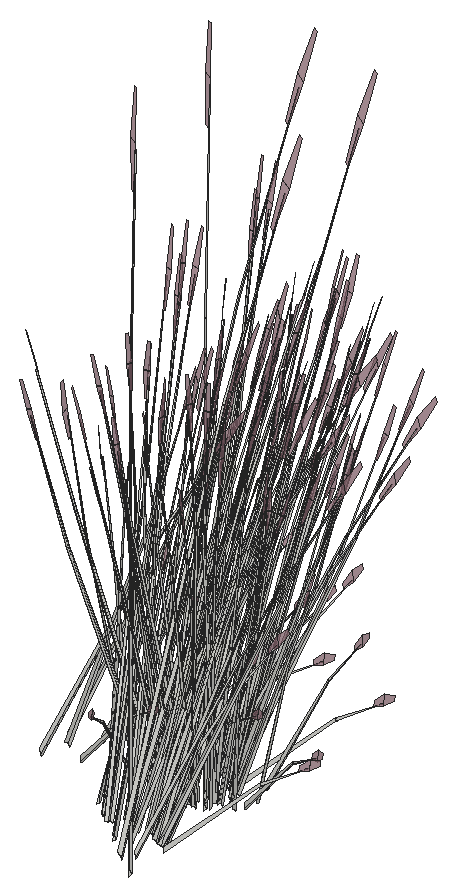
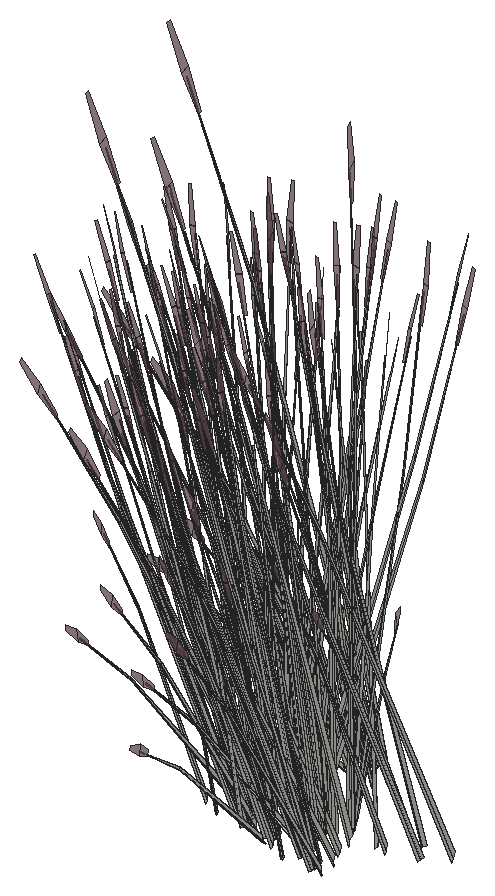
# SketchUp Ruby script. Lengths in inches.
U = 1.inch
M = Sketchup.active_model
def pt(a) = Geom::Point3d.new(a.map { |v| v * U })
def face(e, loops, mat)
  f = e.add_face(loops[0].map { |a| pt(a) })
  loops[1..].each { |l| e.add_face(l.map { |a| pt(a) }).erase! }
  f.material = f.back_material = mat if mat
  f
end
# faces: each face lists its corners as indices into pts; further lists are holes
def faces(e, pts, list, mat = nil) = list.each { |f| face(e, (f[0].is_a?(Array) ? f : [f]).map { |l| l.map { |i| pts[i] } }, mat) }
# xy, xz, yz: faces in a plane at the given z, y or x. An outline is a flat list of corners, or four numbers for a rectangle; further outlines are holes
def ring(l) = l.size == 4 ? [[l[0], l[1]], [l[2], l[1]], [l[2], l[3]], [l[0], l[3]]] : l.each_slice(2).to_a
def flat(e, list, mat, &to3) = list.each { |f| face(e, (f[0].is_a?(Array) ? f : [f]).map { |l| ring(l).map { |u, v| to3.(u, v) } }, mat) }
def xy(e, z, list, mat = nil) = flat(e, list, mat) { |x, y| [x, y, z] }
def xz(e, y, list, mat = nil) = flat(e, list, mat) { |x, z| [x, y, z] }
def yz(e, x, list, mat = nil) = flat(e, list, mat) { |y, z| [x, y, z] }
def lines(e, pts, list) = list.each { |a, b| e.add_line(pt(pts[a]), pt(pts[b])) }
# prism: a flat outline (further loops are holes) pulled along v
def prism(e, loops, v, mat = nil)
  f = face(e, loops, mat); d = Geom::Vector3d.new(v.map { |x| x * U })
  f.pushpull(f.normal.samedirection?(d) ? d.length : -d.length)
end
def box(e, o, s, mat = nil) = prism(e, [[o, [o[0] + s[0], o[1], o[2]], [o[0] + s[0], o[1] + s[1], o[2]], [o[0], o[1] + s[1], o[2]]]], [0, 0, s[2]], mat)
def at(x, y, z, deg = 0) = Geom::Transformation.translation(pt([x, y, z])) * Geom::Transformation.rotation(ORIGIN, Z_AXIS, deg.degrees)
def axes(o, x, y, z) = Geom::Transformation.new([*x, 0, *y, 0, *z, 0, *pt(o).to_a, 1])
def part(name) = M.definitions.add(name)
# library, detail: a bought-in or finely detailed component or shape, given as its bounding box
def library(name, o, s) = part(name).tap { |d| box(d.entities, o, s) }
def detail(e, o, s) = box(e.add_group.entities, o, s)
def put(e, d, t, mat = nil) = e.add_instance(d, t).tap { |i| i.material = mat if mat }
def group(e, t, mat = nil) = e.add_group.tap { |g| g.transformation = t; g.material = mat if mat }.entities
root = M.entities
M.materials.add("LightPink_Translucent").color = [144, 107, 117]
M.materials["LightPink_Translucent"].alpha = 0.75
c1 = part("blade")
p = [[2.15,0.21,22],[0,0.17,0],[0.09,0.45,0],[2.18,0.31,22],[2.29,0.31,22],[0.38,0.45,0],
  [2.48,0.24,33],[2.49,0.24,33],[2.48,0.22,33]]
faces(c1.entities,p,[[0,1,2,3],[4,5,2,3],[6,3,4,7],[8,0,3,6]])
c2 = part("seeds")
p = [[0.3,-0.1,1.38],[-0.01,-0.03,1.59],[-0.01,-0.03,0.03],[0.14,-0.07,-0.07],[0.29,-0.03,3],[0.15,0.01,3.11]]
faces(c2.entities,p,[[0,1,2,3],[1,0,4,5]],"LightPink_Translucent")
c3 = part("blade with seeds")
put(c3.entities,c1,at(0,0,0))
put(c3.entities,c2,axes([2.4,0.25,30.99],[1.5799,-0.05474,1.17369],[-0.12525,1.92788,0.29478],[-0.07173,-0.02425,1.56792]))
put(root,c3,axes([683.69,340.44,268.15],[0.46573,0.38364,-0.47077],[-0.49199,0.33598,-0.36465],[-0.07086,0.19492,0.90078]))
put(root,c3,axes([683.02,333.47,267.91],[0.07381,-0.03447,1.47228],[0.61004,0.22929,-0.13912],[-0.01434,0.19091,0.26054]))
put(root,c3,axes([681.5,338.35,268.13],[0.01693,-0.52814,-0.58968],[0.71285,0.03547,0.07116],[0.07523,-0.22375,0.83415]))
put(root,c3,axes([683.48,340.16,268.19],[0.4402,-0.30062,0.29394],[0.41671,0.34326,-0.37948],[-0.0634,0.1744,0.72609]))
put(root,c3,axes([677.14,338.38,268.13],[0.65035,0.01375,-0.58968],[-0.04368,0.5789,0.07116],[0.27552,0.06109,0.83415]))
put(root,c3,axes([686.43,338.5,266.36],[-0.01777,-0.53759,1.17256],[0.80434,0.13935,0.49647],[-0.19024,0.29416,1.1068]))
put(root,c3,axes([679.15,339.12,267.91],[-0.05883,-0.04999,1.47228],[0.12868,-0.53581,-0.13912],[0.23172,-0.03423,0.26054]))
put(root,c3,axes([676.71,336.8,267.22],[-0.26985,0.01293,1.42242],[0.17902,-0.56047,0.11501],[0.38456,0.03467,0.60807]))
put(root,c3,axes([683.2,340.24,268.48],[0.71502,0.02829,-0.11203],[-0.01954,0.53563,-0.62183],[-0.04967,0.20629,0.94486]))
put(root,c3,axes([684.89,332.08,268.43],[-0.01693,0.52814,-0.65454],[-0.71285,-0.03547,0.07899],[-0.07523,0.22375,0.92591]))
put(root,c3,axes([680.67,342.12,268.19],[-0.10048,-0.4599,0.29394],[0.5744,-0.12144,-0.37948],[0.15428,0.13179,0.72609]))
put(root,c3,axes([685.95,336.23,268.18],[-0.63664,0.26583,-0.10093],[-0.31286,-0.47181,-0.56021],[-0.084,-0.19882,0.85122]))
put(root,c3,axes([685.4,336.26,267.89],[-0.63954,-0.14313,-0.42412],[0.21921,-0.49074,-0.32852],[-0.05864,-0.19758,0.81151]))
put(root,c3,axes([684.22,339.89,267.22],[-0.01592,-0.21915,1.42242],[0.69015,0.14538,0.11501],[-0.04269,0.3123,0.60807]))
put(root,c3,axes([677.7,337.33,268.13],[0.57168,-0.25217,-0.58968],[0.3186,0.51908,0.07116],[0.27622,-0.05897,0.83415]))
put(root,c3,axes([681.05,339.48,267.71],[-0.56218,-0.29666,1.14775],[0.59361,-0.46189,0.49522],[0.18138,0.27836,1.10941]))
put(root,c3,axes([681.79,338.03,267.76],[0.4402,-0.30062,-0.29394],[0.41671,0.34326,0.37948],[0.0634,-0.1744,0.72609]))
put(root,c3,axes([680.11,342.77,267.91],[0.00193,-0.06913,1.47228],[0.55753,-0.30498,-0.13912],[0.19366,0.10886,0.26054]))
put(root,c3,axes([681.96,338.18,267.93],[0.53464,0.0266,0.05337],[-0.01466,0.40172,0.42015],[0.05594,-0.15388,0.64067]))
put(root,c3,axes([684.65,332.82,266.79],[0.01429,-0.29475,1.28107],[0.64291,0.15569,0.17703],[-0.0557,0.31414,0.60492]))
put(root,c3,axes([679.625,336.77,267.91],[0.09028,-0.08697,1.45204],[-0.11555,-0.53348,-0.22964],[0.22652,-0.10115,0.11645]))
put(root,c3,axes([682.49,337.52,267.91],[-0.00628,-0.11364,1.45204],[-0.53042,-0.32843,-0.22964],[0.08201,-0.19909,0.11645]))
put(root,c3,axes([681.79,338.14,267.93],[0.46327,0.38957,0.39842],[-0.49199,0.33598,0.32852],[0.08546,-0.18277,0.82444]))
put(root,c3,axes([685.03,332.25,268.15],[0.46573,0.38364,-0.47077],[-0.49199,0.33598,-0.36465],[-0.07086,0.19492,0.90078]))
put(root,c3,axes([684.82,331.97,268.19],[0.4402,-0.30062,0.29394],[0.41671,0.34326,-0.37948],[-0.0634,0.1744,0.72609]))
put(root,c3,axes([685.76,336.42,268.19],[-0.19614,0.43908,0.29394],[-0.57222,-0.12807,-0.37948],[-0.05247,-0.17678,0.72609]))
put(root,c3,axes([682.33,339.38,268.19],[-0.56631,0.0816,0.29394],[-0.14954,-0.46647,-0.37948],[0.16229,-0.12529,0.72609]))
put(root,c3,axes([687.77,330.3125,266.36],[-0.01777,-0.53759,1.17256],[0.80434,0.13935,0.49647],[-0.19024,0.29416,1.1068]))
put(root,c3,axes([684.71,341.01,268.2],[-0.64106,-0.14927,0.44225],[0.21921,-0.49074,0.36465],[0.03852,0.19299,0.91512]))
put(root,c3,axes([680.7,338.08,267.22],[-0.12114,0.19625,1.42242],[-0.50818,-0.40613,0.11501],[0.22925,-0.25313,0.60807]))
put(root,c3,axes([684.54,341.05,267.93],[-0.47939,0.19405,0.05337],[-0.23464,-0.35385,0.42015],[0.0463,0.15598,0.64067]))
put(root,c3,axes([684.54,332.05,268.48],[0.71502,0.02829,-0.11203],[-0.01954,0.53563,-0.62183],[-0.04967,0.20629,0.94486]))
put(root,c3,axes([680.61,342.36,268.18],[0.38768,-0.48872,-0.10093],[0.56143,0.28156,-0.56021],[0.19516,0.13808,0.85122]))
put(root,c3,axes([682.62,339.43,268.18],[-0.60181,-0.31483,-0.10093],[0.34671,-0.45593,-0.56021],[0.17003,-0.15849,0.85122]))
put(root,c3,axes([685.56,331.7,267.22],[-0.01592,-0.21915,1.42242],[0.69015,0.14538,0.11501],[-0.04269,0.3123,0.60807]))
put(root,c3,axes([681.07,342.12,267.89],[0.64198,-0.13573,-0.42412],[0.1123,0.514,-0.32852],[0.17243,0.1473,0.81151]))
put(root,c3,axes([681.81,341.5,268.19],[-0.37017,-0.35748,0.29394],[0.42268,-0.3384,-0.37948],[0.21476,0.05149,0.72609]))
put(root,c3,axes([684.78,341.12,267.76],[-0.19614,0.43908,-0.29394],[-0.57222,-0.12807,0.37948],[0.05247,0.17678,0.72609]))
put(root,c3,axes([682.15,341.83,267.93],[-0.03276,0.43418,0.05337],[-0.49468,-0.0119,0.42015],[0.18949,0.04543,0.64067]))
put(root,c3,axes([682.19,341.6875,267.93],[-0.47971,0.37622,0.39842],[-0.41372,-0.39954,0.32852],[0.22506,0.0694,0.82444]))
put(root,c3,axes([682.32,339.05,267.89],[-0.16713,-0.52135,-0.42412],[0.63294,-0.0912,-0.32852],[0.18138,-0.14003,0.81151]))
put(root,c3,axes([683.4375,341.74,267.26],[-0.12452,-0.47997,-0.02898],[0.58854,-0.11034,-0.1314],[0.1229,0.03043,0.43341]))
put(root,c3,axes([682.42,340.5,268.19],[-0.54068,-0.15928,0.29394],[0.1577,-0.46469,-0.37948],[0.21769,-0.04261,0.72609]))
put(root,c3,axes([685.93,336.02,267.93],[0.47939,-0.19405,0.05337],[0.23464,0.35385,0.42015],[-0.0463,-0.15598,0.64067]))
put(root,c3,axes([684.375,341.89,267.91],[0.08247,0.09194,1.45204],[0.66552,0.03612,-0.22964],[0.06692,0.20277,0.11645]))
put(root,c3,axes([686.05,332.83,268.2],[-0.64106,-0.14927,0.44225],[0.21921,-0.49074,0.36465],[0.03852,0.19299,0.91512]))
put(root,c3,axes([685.76,336.06,267.93],[0.64106,0.14927,0.39842],[-0.21921,0.49074,0.32852],[-0.03852,-0.19299,0.82444]))
put(root,c3,axes([685.88,332.86,267.93],[-0.47939,0.19405,0.05337],[-0.23464,-0.35385,0.42015],[0.0463,0.15598,0.64067]))
put(root,c3,axes([682.84,339.31,267.93],[0.44663,0.24013,0.05337],[-0.26003,0.34195,0.42015],[0.14319,-0.11055,0.64067]))
put(root,c3,axes([684.72,340.65,268.19],[0.19614,-0.43908,0.29394],[0.57222,0.12807,-0.37948],[0.05247,0.17678,0.72609]))
put(root,c3,axes([682.72,339.21,267.93],[0.16135,0.52549,0.39842],[-0.63294,0.0912,0.32852],[0.18654,-0.12359,0.82444]))
put(root,c3,axes([681.01,340.77,267.22],[-0.24166,-0.09837,1.42242],[0.50011,-0.41269,0.11501],[0.3117,0.18617,0.60807]))
put(root,c3,axes([684.84,340.72,268.13],[0.31051,0.46426,-0.58968],[-0.63919,0.25873,0.07116],[0.07261,0.22432,0.83415]))
put(root,c3,axes([684.1,339.29,267.91],[-0.08498,-0.00434,1.47228],[-0.35287,-0.46464,-0.13912],[0.14171,-0.15278,0.26054]))
put(root,c3,axes([682.79,339.11,267.76],[0.56631,-0.0816,-0.29394],[0.14954,0.46647,0.37948],[0.16229,-0.12529,0.72609]))
put(root,c3,axes([682.34,339.26,268.13],[0.33983,-0.45051,-0.58968],[0.59551,0.32017,0.07116],[0.20291,-0.16322,0.83415]))
put(root,c3,axes([682.91,340.64,267.93],[0.23895,0.38931,0.05337],[-0.43573,0.19055,0.42015],[0.19208,-0.0376,0.64067]))
put(root,c3,axes([686.12,332.93,267.76],[-0.19614,0.43908,-0.29394],[-0.57222,-0.12807,0.37948],[0.05247,0.17678,0.72609]))
put(root,c3,axes([682.33,341.6875,267.76],[0.37017,0.35748,-0.29394],[-0.42268,0.3384,0.37948],[0.21476,0.05149,0.72609]))
put(root,c3,axes([681.91,341.73,268.18],[0.03484,-0.58066,-0.10093],[0.65957,0.01587,-0.56021],[0.25402,0.04034,0.85122]))
put(root,c3,axes([682.65,340.65,268.18],[-0.32734,-0.51701,-0.10093],[0.58097,-0.25407,-0.56021],[0.24483,-0.06821,0.85122]))
put(root,c3,axes([685.49,342.22,268.6875],[0.44958,-0.32756,-0.05385],[0.41194,0.35875,-0.24415],[0.029,0.10165,0.8053]))
put(root,c3,axes([682.86,340.51,267.93],[-0.18381,0.5206,0.39842],[-0.60429,-0.17802,0.32852],[0.23764,-0.03129,0.82444]))
put(root,c3,axes([685.07,340.81,267.89],[0.63954,0.14313,-0.42412],[-0.21921,0.49074,-0.32852],[0.05864,0.19758,0.81151]))
put(root,c3,axes([684.53,340.84,268.18],[0.63664,-0.26583,-0.10093],[0.31286,0.47181,-0.56021],[0.084,0.19882,0.85122]))
put(root,c3,axes([687.27,336.83,268.18],[-0.71502,-0.02829,-0.10093],[0.01954,-0.53563,-0.56021],[0.04967,-0.20629,0.85122]))
put(root,c3,axes([685.72,333.71,267.91],[0.08247,0.09194,1.45204],[0.66552,0.03612,-0.22964],[0.06692,0.20277,0.11645]))
put(root,c3,axes([682.48,341.38,267.91],[0.13956,-0.00966,1.45204],[0.38281,-0.44358,-0.22964],[0.24825,0.05855,0.11645]))
put(root,c3,axes([682.62,340.21,267.89],[0.17625,-0.51936,-0.42412],[0.60429,0.17802,-0.32852],[0.2433,-0.04762,0.81151]))
put(root,c3,axes([686.06,332.46,268.19],[0.19614,-0.43908,0.29394],[0.57222,0.12807,-0.37948],[0.05247,0.17678,0.72609]))
put(root,c3,axes([686.99,336.91,268.19],[-0.4402,0.30062,0.29394],[-0.41671,-0.34326,-0.37948],[0.0634,-0.1744,0.72609]))
put(root,c3,axes([686.78,336.63,267.89],[-0.46573,-0.38364,-0.42412],[0.49199,-0.33598,-0.32852],[0.07086,-0.19492,0.81151]))
put(root,c3,axes([682.99,340.45,267.76],[0.54068,0.15928,-0.29394],[-0.1577,0.46469,0.37948],[0.21769,-0.04261,0.72609]))
put(root,c3,axes([686.18,332.53,268.13],[0.31051,0.46426,-0.58968],[-0.63919,0.25873,0.07116],[0.07261,0.22432,0.83415]))
put(root,c3,axes([681.94,341.45,268.13],[0.65035,0.01375,-0.58968],[-0.04368,0.5789,0.07116],[0.27552,0.06109,0.83415]))
put(root,c3,axes([686.83,334.03,268.6875],[0.44958,-0.32756,-0.05385],[0.41194,0.35875,-0.24415],[0.029,0.10165,0.8053]))
put(root,c3,axes([683.95,342.19,267.91],[-0.05883,-0.04999,1.47228],[0.12868,-0.53581,-0.13912],[0.23172,-0.03423,0.26054]))
put(root,c3,axes([686.31,340.9,267.93],[-0.64708,0.13103,0.39842],[-0.1123,-0.514,0.32852],[0.15218,0.15149,0.82444]))
put(root,c3,axes([681.52,339.87,267.22],[-0.26985,0.01293,1.42242],[0.17902,-0.56047,0.11501],[0.38456,0.03467,0.60807]))
put(root,c3,axes([686.18,341,267.93],[-0.29569,0.36271,0.05337],[-0.42107,-0.21117,0.42015],[0.13613,0.11629,0.64067]))
put(root,c3,axes([685.44,339.8,267.22],[-0.14872,-0.18332,1.42242],[0.6872,-0.15433,0.11501],[0.15531,0.28779,0.60807]))
put(root,c3,axes([686.41,332.625,267.89],[0.63954,0.14313,-0.42412],[-0.21921,0.49074,-0.32852],[0.05864,0.19758,0.81151]))
put(root,c3,axes([685.87,332.65,268.18],[0.63664,-0.26583,-0.10093],[0.31286,0.47181,-0.56021],[0.084,0.19882,0.85122]))
put(root,c3,axes([682.5,340.4,268.13],[0.57168,-0.25217,-0.58968],[0.3186,0.51908,0.07116],[0.27622,-0.05897,0.83415]))
put(root,c3,axes([684.42,339.84,267.91],[0.09028,-0.08697,1.45204],[-0.11555,-0.53348,-0.22964],[0.22652,-0.10115,0.11645]))
put(root,c3,axes([686.09,340.58,268.19],[-0.10048,-0.4599,0.29394],[0.5744,-0.12144,-0.37948],[0.15428,0.13179,0.72609]))
put(root,c3,axes([686.48,337.93,267.71],[-0.56218,-0.29666,1.14775],[0.59361,-0.46189,0.49522],[0.18138,0.27836,1.10941]))
put(root,c3,axes([687.22,336.49,267.76],[0.4402,-0.30062,-0.29394],[0.41671,0.34326,0.37948],[0.0634,-0.1744,0.72609]))
put(root,c3,axes([685.53,341.22,267.91],[0.00193,-0.06913,1.47228],[0.55753,-0.30498,-0.13912],[0.19366,0.10886,0.26054]))
put(root,c3,axes([687.39,336.64,267.93],[0.53464,0.0266,0.05337],[-0.01466,0.40172,0.42015],[0.05594,-0.15388,0.64067]))
put(root,c3,axes([687.22,336.6,267.93],[0.46327,0.38957,0.39842],[-0.49199,0.33598,0.32852],[0.08546,-0.18277,0.82444]))
put(root,c3,axes([687.65,332.71,267.93],[-0.64708,0.13103,0.39842],[-0.1123,-0.514,0.32852],[0.15218,0.15149,0.82444]))
put(root,c3,axes([687.52,332.81,267.93],[-0.29569,0.36271,0.05337],[-0.42107,-0.21117,0.42015],[0.13613,0.11629,0.64067]))
put(root,c3,axes([686.77,331.61,267.22],[-0.14872,-0.18332,1.42242],[0.6872,-0.15433,0.11501],[0.15531,0.28779,0.60807]))
put(root,c3,axes([687.75,337.84,268.19],[-0.56631,0.0816,0.29394],[-0.14954,-0.46647,-0.37948],[0.16229,-0.12529,0.72609]))
put(root,c3,axes([687.43,332.39,268.19],[-0.10048,-0.4599,0.29394],[0.5744,-0.12144,-0.37948],[0.15428,0.13179,0.72609]))
put(root,c3,axes([686.04,340.82,268.18],[0.38768,-0.48872,-0.10093],[0.56143,0.28156,-0.56021],[0.19516,0.13808,0.85122]))
put(root,c3,axes([688.05,337.88,268.18],[-0.60181,-0.31483,-0.10093],[0.34671,-0.45593,-0.56021],[0.17003,-0.15849,0.85122]))
put(root,c3,axes([687.82,329.75,267.71],[-0.56218,-0.29666,1.14775],[0.59361,-0.46189,0.49522],[0.18138,0.27836,1.10941]))
put(root,c3,axes([686.87,333.04,267.91],[0.00193,-0.06913,1.47228],[0.55753,-0.30498,-0.13912],[0.19366,0.10886,0.26054]))
put(root,c3,axes([686.5,340.58,267.89],[0.64198,-0.13573,-0.42412],[0.1123,0.514,-0.32852],[0.17243,0.1473,0.81151]))
put(root,c3,axes([687.24,339.96,268.19],[-0.37017,-0.35748,0.29394],[0.42268,-0.3384,-0.37948],[0.21476,0.05149,0.72609]))
put(root,c3,axes([687.57,340.28,267.93],[-0.03276,0.43418,0.05337],[-0.49468,-0.0119,0.42015],[0.18949,0.04543,0.64067]))
put(root,c3,axes([687.62,340.14,267.93],[-0.47971,0.37622,0.39842],[-0.41372,-0.39954,0.32852],[0.22506,0.0694,0.82444]))
put(root,c3,axes([687.75,337.51,267.89],[-0.16713,-0.52135,-0.42412],[0.63294,-0.0912,-0.32852],[0.18138,-0.14003,0.81151]))
put(root,c3,axes([688.86,340.2,267.26],[-0.12452,-0.47997,-0.02898],[0.58854,-0.11034,-0.1314],[0.1229,0.03043,0.43341]))
put(root,c3,axes([687.84,338.96,268.19],[-0.54068,-0.15928,0.29394],[0.1577,-0.46469,-0.37948],[0.21769,-0.04261,0.72609]))
put(root,c3,axes([688.27,337.77,267.93],[0.44663,0.24013,0.05337],[-0.26003,0.34195,0.42015],[0.14319,-0.11055,0.64067]))
put(root,c3,axes([687.38,332.63,268.18],[0.38768,-0.48872,-0.10093],[0.56143,0.28156,-0.56021],[0.19516,0.13808,0.85122]))
put(root,c3,axes([688.14,337.67,267.93],[0.16135,0.52549,0.39842],[-0.63294,0.0912,0.32852],[0.18654,-0.12359,0.82444]))
put(root,c3,axes([686.43,339.23,267.22],[-0.24166,-0.09837,1.42242],[0.50011,-0.41269,0.11501],[0.3117,0.18617,0.60807]))
put(root,c3,axes([689.53,337.75,267.91],[-0.08498,-0.00434,1.47228],[-0.35287,-0.46464,-0.13912],[0.14171,-0.15278,0.26054]))
put(root,c3,axes([687.84,332.39,267.89],[0.64198,-0.13573,-0.42412],[0.1123,0.514,-0.32852],[0.17243,0.1473,0.81151]))
put(root,c3,axes([688.22,337.57,267.76],[0.56631,-0.0816,-0.29394],[0.14954,0.46647,0.37948],[0.16229,-0.12529,0.72609]))
put(root,c3,axes([687.77,337.72,268.13],[0.33983,-0.45051,-0.58968],[0.59551,0.32017,0.07116],[0.20291,-0.16322,0.83415]))
put(root,c3,axes([688.33,339.1,267.93],[0.23895,0.38931,0.05337],[-0.43573,0.19055,0.42015],[0.19208,-0.0376,0.64067]))
put(root,c3,axes([687.76,340.15,267.76],[0.37017,0.35748,-0.29394],[-0.42268,0.3384,0.37948],[0.21476,0.05149,0.72609]))
put(root,c3,axes([687.34,340.1875,268.18],[0.03484,-0.58066,-0.10093],[0.65957,0.01587,-0.56021],[0.25402,0.04034,0.85122]))
put(root,c3,axes([688.07,339.11,268.18],[-0.32734,-0.51701,-0.10093],[0.58097,-0.25407,-0.56021],[0.24483,-0.06821,0.85122]))
put(root,c3,axes([688.91,332.09,267.93],[-0.03276,0.43418,0.05337],[-0.49468,-0.0119,0.42015],[0.18949,0.04543,0.64067]))
put(root,c3,axes([688.29,338.96,267.93],[-0.18381,0.5206,0.39842],[-0.60429,-0.17802,0.32852],[0.23764,-0.03129,0.82444]))
put(root,c3,axes([688.96,331.96,267.93],[-0.47971,0.37622,0.39842],[-0.41372,-0.39954,0.32852],[0.22506,0.0694,0.82444]))
put(root,c3,axes([687.91,339.84,267.91],[0.13956,-0.00966,1.45204],[0.38281,-0.44358,-0.22964],[0.24825,0.05855,0.11645]))
put(root,c3,axes([688.04,338.67,267.89],[0.17625,-0.51936,-0.42412],[0.60429,0.17802,-0.32852],[0.2433,-0.04762,0.81151]))
put(root,c3,axes([688.41,338.91,267.76],[0.54068,0.15928,-0.29394],[-0.1577,0.46469,0.37948],[0.21769,-0.04261,0.72609]))
put(root,c3,axes([687.77,331.04,267.22],[-0.24166,-0.09837,1.42242],[0.50011,-0.41269,0.11501],[0.3117,0.18617,0.60807]))
put(root,c3,axes([687.37,339.91,268.13],[0.65035,0.01375,-0.58968],[-0.04368,0.5789,0.07116],[0.27552,0.06109,0.83415]))
put(root,c3,axes([689.1,331.96,267.76],[0.37017,0.35748,-0.29394],[-0.42268,0.3384,0.37948],[0.21476,0.05149,0.72609]))
put(root,c3,axes([689.375,340.65,267.91],[-0.05883,-0.04999,1.47228],[0.12868,-0.53581,-0.13912],[0.23172,-0.03423,0.26054]))
put(root,c3,axes([686.94,338.33,267.22],[-0.26985,0.01293,1.42242],[0.17902,-0.56047,0.11501],[0.38456,0.03467,0.60807]))
put(root,c3,axes([687.93,338.86,268.13],[0.57168,-0.25217,-0.58968],[0.3186,0.51908,0.07116],[0.27622,-0.05897,0.83415]))
put(root,c3,axes([689.25,331.65,267.91],[0.13956,-0.00966,1.45204],[0.38281,-0.44358,-0.22964],[0.24825,0.05855,0.11645]))
put(root,c3,axes([689.85,338.3,267.91],[0.09028,-0.08697,1.45204],[-0.11555,-0.53348,-0.22964],[0.22652,-0.10115,0.11645]))
put(root,c3,axes([688.71,331.72,268.13],[0.65035,0.01375,-0.58968],[-0.04368,0.5789,0.07116],[0.27552,0.06109,0.83415]))
